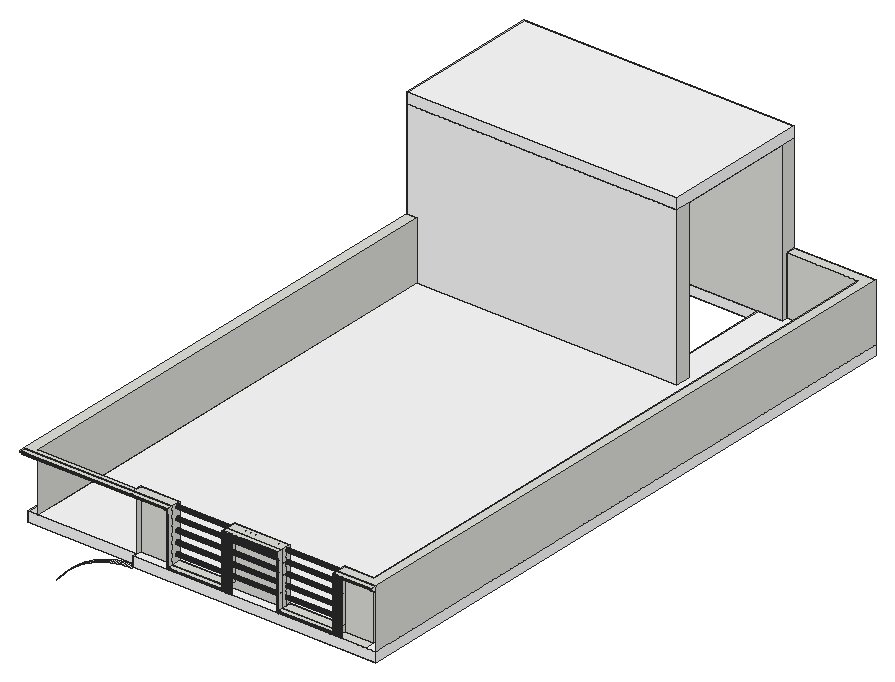
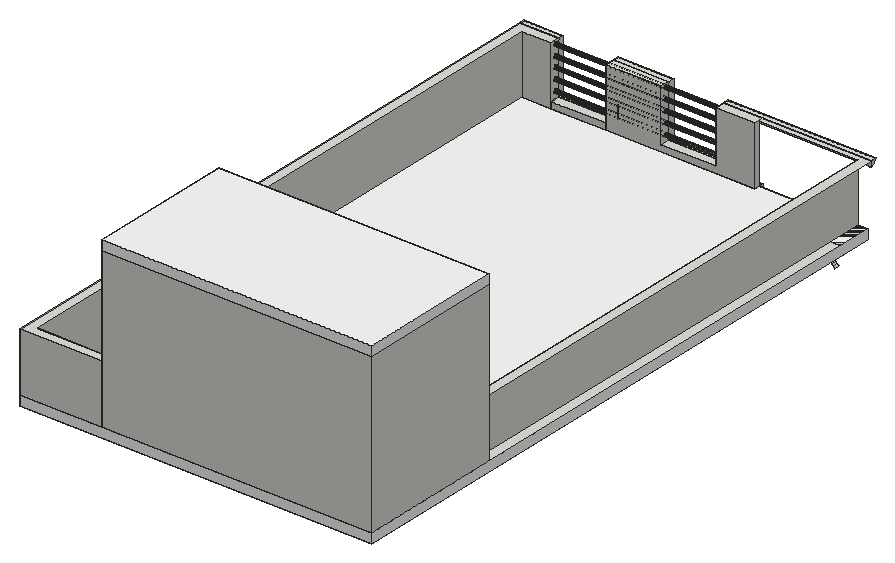
# SketchUp Ruby script. Lengths in inches.
U = 1.inch
M = Sketchup.active_model
def pt(a) = Geom::Point3d.new(a.map { |v| v * U })
def face(e, loops, mat)
  f = e.add_face(loops[0].map { |a| pt(a) })
  loops[1..].each { |l| e.add_face(l.map { |a| pt(a) }).erase! }
  f.material = f.back_material = mat if mat
  f
end
# faces: each face lists its corners as indices into pts; further lists are holes
def faces(e, pts, list, mat = nil) = list.each { |f| face(e, (f[0].is_a?(Array) ? f : [f]).map { |l| l.map { |i| pts[i] } }, mat) }
# xy, xz, yz: faces in a plane at the given z, y or x. An outline is a flat list of corners, or four numbers for a rectangle; further outlines are holes
def ring(l) = l.size == 4 ? [[l[0], l[1]], [l[2], l[1]], [l[2], l[3]], [l[0], l[3]]] : l.each_slice(2).to_a
def flat(e, list, mat, &to3) = list.each { |f| face(e, (f[0].is_a?(Array) ? f : [f]).map { |l| ring(l).map { |u, v| to3.(u, v) } }, mat) }
def xy(e, z, list, mat = nil) = flat(e, list, mat) { |x, y| [x, y, z] }
def xz(e, y, list, mat = nil) = flat(e, list, mat) { |x, z| [x, y, z] }
def yz(e, x, list, mat = nil) = flat(e, list, mat) { |y, z| [x, y, z] }
def lines(e, pts, list) = list.each { |a, b| e.add_line(pt(pts[a]), pt(pts[b])) }
# prism: a flat outline (further loops are holes) pulled along v
def prism(e, loops, v, mat = nil)
  f = face(e, loops, mat); d = Geom::Vector3d.new(v.map { |x| x * U })
  f.pushpull(f.normal.samedirection?(d) ? d.length : -d.length)
end
def box(e, o, s, mat = nil) = prism(e, [[o, [o[0] + s[0], o[1], o[2]], [o[0] + s[0], o[1] + s[1], o[2]], [o[0], o[1] + s[1], o[2]]]], [0, 0, s[2]], mat)
def at(x, y, z, deg = 0) = Geom::Transformation.translation(pt([x, y, z])) * Geom::Transformation.rotation(ORIGIN, Z_AXIS, deg.degrees)
def axes(o, x, y, z) = Geom::Transformation.new([*x, 0, *y, 0, *z, 0, *pt(o).to_a, 1])
def part(name) = M.definitions.add(name)
# library, detail: a bought-in or finely detailed component or shape, given as its bounding box
def library(name, o, s) = part(name).tap { |d| box(d.entities, o, s) }
def detail(e, o, s) = box(e.add_group.entities, o, s)
def put(e, d, t, mat = nil) = e.add_instance(d, t).tap { |i| i.material = mat if mat }
def group(e, t, mat = nil) = e.add_group.tap { |g| g.transformation = t; g.material = mat if mat }.entities
root = M.entities
M.materials.add("Leather White 002 15.0cm").color = [255, 255, 255]
M.materials.add("Manhattan Creative Coating ML 1016B 24.75cm").color = [255, 255, 255]
M.materials.add("Napura - nsi3013 29.32cm").color = [255, 255, 255]
M.materials.add("Steel Blurry").color = [182, 192, 192]
M.materials.add("T8600 Mosaic plaster 1019 34.05cm").color = [255, 255, 255]
c1 = part("Vertical post")
prism(c1.entities,[[[0.67,1.9375,0],[0.73,1.96,0],[0.99,2,0],[1.25,1.97,0],[1.49,1.87,0],[1.7,1.72,0],[1.86,1.51,0],[1.96,1.27,0],[2,1.01,0],[1.97,0.75,0],[1.87,0.51,0],[1.72,0.3,0],[1.51,0.14,0],[1.27,0.04,0],[1.01,0,0],[0.75,0.03,0],[0.67,0.0625,0],[0.51,0.13,0],[0.3,0.28,0],[0.14,0.49,0],[0.04,0.73,0],[0,0.99,0],[0.03,1.25,0],[0.13,1.49,0],[0.28,1.7,0],[0.49,1.86,0]]],[0,0,101.21])
xy(root,373.99,[[192.8125,53.93,213,54.62]])
xy(root,378,[[66.79,50.93,158.4,56.93],[158.4,50.93,192,56.93],[210,50.93,210,428.93,165.875,428.93,165.875,434.93,216,434.93,216,50.93],[192,50.93,210,56.93],[0,53.93,6,74.93],
  [0,74.93,6,344.93],[0,344.93,0,434.93,165.875,434.93,165.875,425.93,9,425.93,9,353.93,165.875,353.93,165.875,344.93]])
xy(root,378.5,[[87.54,50.68,127.65,50.93],[155.15,50.68,195.25,50.93]],"T8600 Mosaic plaster 1019 34.05cm")
xy(root,379.42,[[88.46,49.9,88.47,50,126.72,50,126.73,49.9],[156.0625,49.9,156.07,50,194.33,50,194.33,49.9],[88.47,50,88.46,50.09,126.73,50.09,126.72,50],[156.07,50,194.33,50.09]],"T8600 Mosaic plaster 1019 34.05cm")
xy(root,379.54,[[88.59,49.77,126.61,49.9],[156.1875,49.77,194.21,49.9]],"T8600 Mosaic plaster 1019 34.05cm")
xy(root,381.5,[[90.54,47.57,124.65,47.85],[158.15,47.57,192.25,47.85]])
xy(root,381.75,[[90.79,47.57,124.4,50.93],[158.4,47.57,192,50.93],[90.79,50.93,124.4,56.93],[158.4,50.93,192,56.93]])
xy(root,410.75,[[0,50.68,87.54,50.93],[127.65,50.68,127.65,50.93,155.15,50.68],[155.15,50.68,127.65,50.93,155.15,50.93],[195.25,50.68,216,50.93]],"T8600 Mosaic plaster 1019 34.05cm")
xy(root,411.67,[[0,49.9,0,50,88.47,50,88.46,49.9],[126.73,49.9,126.72,50,156.07,50,156.0625,49.9],[194.33,49.9,216,50],[0,50,0,50.09,88.46,50.09,88.47,50],[126.72,50,126.73,50.09,156.07,50.09,156.07,50],
  [194.33,50,216,50.09]],"T8600 Mosaic plaster 1019 34.05cm")
xy(root,411.79,[[0,49.77,88.59,49.9],[126.61,49.77,156.1875,49.9],[194.21,49.77,216,49.9]],"T8600 Mosaic plaster 1019 34.05cm")
xy(root,413.75,[[0,47.57,90.54,47.85],[124.65,47.57,158.15,47.85],[192.25,47.57,216,47.85]])
xy(root,414,[[0,47.57,90.79,50.93],[124.4,47.57,158.4,50.93],[192,47.57,216,50.93],[0,50.93,66.79,50.93,66.79,53.93,6,53.93,6,344.93,0,344.93],[66.79,50.93,90.79,56.93],
  [124.4,50.93,158.4,56.93],[192,50.93,216,50.93,216,434.93,165.875,434.93,165.875,428.93,210,428.93,210,56.93,192,56.93]])
xy(root,474.5625,[[0,344.93,165.875,353.93],[0,353.93,9,425.93],[9,353.93,165.875,425.93],[0,425.93,165.875,434.93]])
xy(root,481,[[0,344.93,165.875,434.93]],"Napura - nsi3013 29.32cm")
xz(root,47.57,[[90.54,381.5,124.65,381.5,124.65,413.75,158.15,413.75,158.15,381.5,192.25,381.5,192.25,413.75,216,413.75,216,414,192,414,192,381.75,158.4,381.75,158.4,414,124.4,414,124.4,381.75,90.79,381.75,90.79,414,0,414,0,413.75,90.54,413.75]],"T8600 Mosaic plaster 1019 34.05cm")
xz(root,47.85,[[90.34,381.29,124.85,381.29,124.85,413.54,157.94,413.54,157.94,381.29,192.46,381.29,192.46,413.54,216,413.54,216,413.75,192.25,413.75,192.25,381.5,158.15,381.5,158.15,413.75,124.65,413.75,124.65,381.5,90.54,381.5,90.54,413.75,0,413.75,0,413.54,90.34,413.54]],"T8600 Mosaic plaster 1019 34.05cm")
xz(root,49.9,[[88.46,379.42,126.73,379.42,126.73,411.67,156.0625,411.67,156.0625,379.42,194.33,379.42,194.33,411.67,216,411.67,216,411.79,194.21,411.79,194.21,379.54,156.1875,379.54,156.1875,411.79,126.61,411.79,126.61,379.54,88.59,379.54,88.59,411.79,0,411.79,0,411.67,88.46,411.67]],"T8600 Mosaic plaster 1019 34.05cm")
xz(root,50.68,[[87.54,378.5,127.65,378.5,127.65,410.75,155.15,410.75,155.15,378.5,195.25,378.5,195.25,410.75,216,410.75,216,411,195,411,195,378.75,155.4,378.75,155.4,411,127.4,411,127.4,378.75,87.79,378.75,87.79,411,0,411,0,410.75,87.54,410.75],[87.79,378.75,127.4,378.75,127.3,378.85,87.89,378.85],[87.79,378.75,87.89,378.85,87.89,411.1,87.79,411],[127.4,378.75,127.4,411,127.3,411.1,127.3,378.85],[155.4,378.75,155.49,378.85,155.49,411.1,155.4,411],
  [155.4,378.75,195,378.75,194.9,378.85,155.49,378.85],[195,378.75,195,411,194.9,411.1,194.9,378.85],[0,411,87.79,411,87.89,411.1,0,411.1],[127.4,411,155.4,411,155.49,411.1,127.3,411.1],[195,411,216,411,216,411.1,194.9,411.1]],"T8600 Mosaic plaster 1019 34.05cm")
xz(root,50.93,[[87.54,378.5,127.65,378.5,127.65,410.75,155.15,410.75,155.15,378.5,195.25,378.5,195.25,410.75,216,410.75,216,414,192,414,192,381.75,158.4,381.75,158.4,414,124.4,414,124.4,381.75,90.79,381.75,90.79,414,0,414,0,410.75,87.54,410.75]])
xz(root,56.93,[[66.79,378,66.79,414,90.79,414,90.79,381.75,124.4,381.75,124.4,414,158.4,414,158.4,378],[158.4,378,192,381.75],[192,378,210,414]])
xz(root,344.93,[[0,378,6,414]])
xz(root,344.93,[[6,378,165.875,378,165.875,474.5625,0,474.5625,0,414,6,414],[0,474.5625,165.875,481]],"Napura - nsi3013 29.32cm")
xz(root,353.93,[[9,378,165.875,474.5625]])
xz(root,425.93,[[9,378,165.875,474.5625]])
xz(root,428.93,[[165.875,378,210,414]])
xz(root,434.93,[[0,378,165.875,474.5625],[165.875,378,216,414]])
xz(root,434.93,[[0,474.5625,165.875,481]],"Napura - nsi3013 29.32cm")
yz(root,0,[[344.93,378,434.93,474.5625],[50.68,410.75,50.68,411.1,50.62,411.28,50.57,411.37,50.51,411.45,50.37,411.57,50.28,411.62,50.1875,411.65,50.09,411.67,49.9,411.67,49.9,411.79,49.77,411.79,49.67,411.8,49.57,411.8125,49.48,411.84,49.38,411.88,49.3,411.93,49.21,411.99,49.07,412.13,48.97,412.31,48.93,412.4,48.91,412.5,48.875,412.625,48.83,412.75,48.77,412.87,48.7,412.98,48.625,413.08,48.54,413.18,48.4375,413.27,48.33,413.34,48.22,413.41,48.1,413.47,47.98,413.51,47.85,413.54,47.85,413.75,47.57,413.75,47.57,414,50.93,414,50.93,410.75]])
yz(root,0,[[344.93,474.5625,434.93,481]],"Napura - nsi3013 29.32cm")
yz(root,6,[[53.93,378,344.93,414]])
yz(root,9,[[353.93,378,425.93,474.5625]])
yz(root,66.79,[[50.93,371.45,53.93,378],[53.93,378,56.93,414]])
yz(root,87.54,[[50.68,378.5,50.93,410.75]],"T8600 Mosaic plaster 1019 34.05cm")
yz(root,88.59,[[49.77,379.54,49.67,379.55,49.67,411.8,49.77,411.79],[49.77,379.54,49.9,411.79]],"T8600 Mosaic plaster 1019 34.05cm")
yz(root,90.54,[[47.57,381.5,47.85,413.75]])
yz(root,90.79,[[47.57,381.75,50.93,414],[50.93,381.75,56.93,414]])
yz(root,124.4,[[47.57,381.75,50.93,414],[50.93,381.75,56.93,414]])
yz(root,124.65,[[47.57,381.5,47.85,413.75]])
yz(root,126.61,[[49.77,379.54,49.9,411.79]],"T8600 Mosaic plaster 1019 34.05cm")
yz(root,127.65,[[50.68,378.5,50.93,410.75]],"T8600 Mosaic plaster 1019 34.05cm")
yz(root,155.15,[[50.68,378.5,50.93,410.75]],"T8600 Mosaic plaster 1019 34.05cm")
yz(root,156.07,[[50,379.42,50.09,411.67]],"T8600 Mosaic plaster 1019 34.05cm")
yz(root,156.1875,[[49.77,379.54,49.9,411.79]],"T8600 Mosaic plaster 1019 34.05cm")
yz(root,158.15,[[47.57,381.5,47.85,413.75]])
yz(root,158.4,[[53.93,378,56.93,381.75],[47.57,381.75,50.93,414],[50.93,381.75,53.93,414],[53.93,381.75,56.93,414]])
yz(root,165.875,[[344.93,378,353.93,474.5625],[425.93,378,428.93,378,428.93,414,434.93,414,434.93,474.5625,425.93,474.5625],[428.93,378,434.93,414]])
yz(root,165.875,[[344.93,474.5625,434.93,481]],"Napura - nsi3013 29.32cm")
yz(root,192,[[53.93,378,56.93,381.75],[47.57,381.75,50.93,414],[50.93,381.75,56.93,414]])
yz(root,192.25,[[47.57,381.5,47.85,413.75]])
yz(root,194.21,[[49.77,379.54,49.9,411.79]],"T8600 Mosaic plaster 1019 34.05cm")
yz(root,194.33,[[49.9,379.42,50,411.67],[50,379.42,50.09,411.67]],"T8600 Mosaic plaster 1019 34.05cm")
yz(root,195.25,[[50.68,378.5,50.93,410.75]],"T8600 Mosaic plaster 1019 34.05cm")
yz(root,210,[[56.93,378,428.93,414]])
yz(root,216,[[50.93,378,434.93,414]])
yz(root,216,[[50.68,410.75,50.93,410.75,50.93,414,47.57,414,47.57,413.75,47.85,413.75,47.85,413.54,47.98,413.51,48.1,413.47,48.22,413.41,48.33,413.34,48.4375,413.27,48.54,413.18,48.625,413.08,48.7,412.98,48.77,412.87,48.83,412.75,48.875,412.625,48.91,412.5,48.93,412.4,48.97,412.31,49.07,412.13,49.21,411.99,49.3,411.93,49.38,411.88,49.48,411.84,49.57,411.8125,49.67,411.8,49.77,411.79,49.9,411.79,49.9,411.67,50.09,411.67,50.1875,411.65,50.28,411.62,50.37,411.57,50.51,411.45,50.57,411.37,50.62,411.28,50.68,411.1]],"T8600 Mosaic plaster 1019 34.05cm")
p = [[20.99,50.93,349.89],[20.21,50.93,348.93],[20.21,53.93,348.93],[20.99,53.93,349.89],[21.79,50.93,350.84],[21.79,53.93,350.84],
  [22.62,50.93,351.78],[22.62,53.93,351.78],[23.46,50.93,352.7],[23.46,53.93,352.7],[24.32,50.93,353.59],[24.32,53.93,353.59],
  [25.2,50.93,354.47],[25.2,53.93,354.47],[26.1,50.93,355.34],[26.1,53.93,355.34],[27.02,50.93,356.18],[27.02,53.93,356.18],
  [27.95,50.93,357],[27.95,53.93,357],[28.9,50.93,357.81],[28.9,53.93,357.81],[29.87,50.93,358.59],[29.87,53.93,358.59],
  [30.85,50.93,359.35],[30.85,53.93,359.35],[31.85,50.93,360.09],[31.85,53.93,360.09],[32.87,50.93,360.82],[32.87,53.93,360.82],
  [33.9,50.93,361.52],[33.9,53.93,361.52],[34.94,50.93,362.19],[34.94,53.93,362.19],[36,50.93,362.85],[36,53.93,362.85],
  [37.07,50.93,363.48],[37.07,53.93,363.48],[38.16,50.93,364.1],[38.16,53.93,364.1],[39.25,50.93,364.68],[39.25,53.93,364.68],
  [40.36,50.93,365.25],[40.36,53.93,365.25],[41.48,50.93,365.79],[41.48,53.93,365.79],[42.62,50.93,366.31],[42.62,53.93,366.31],
  [43.76,50.93,366.8],[43.76,53.93,366.8],[44.91,50.93,367.27],[44.91,53.93,367.27],[46.07,50.93,367.72],[46.07,53.93,367.72],
  [47.24,50.93,368.14],[47.24,53.93,368.14],[48.42,50.93,368.54],[48.42,53.93,368.54],[49.61,50.93,368.91],[49.61,53.93,368.91],
  [50.81,50.93,369.26],[50.81,53.93,369.26],[52.01,50.93,369.58],[52.01,53.93,369.58],[53.22,50.93,369.88],[53.22,53.93,369.88],
  [54.43,50.93,370.15],[54.43,53.93,370.15],[55.66,50.93,370.4],[55.66,53.93,370.4],[56.88,50.93,370.62],[56.88,53.93,370.62],
  [58.11,50.93,370.8125],[58.11,53.93,370.8125],[59.34,50.93,370.98],[59.34,53.93,370.98],[60.58,50.93,371.12],[60.58,53.93,371.12],
  [61.82,50.93,371.24],[61.82,53.93,371.24],[63.0625,50.93,371.33],[63.0625,53.93,371.33],[64.31,50.93,371.4],[64.31,53.93,371.4],
  [65.55,50.93,371.44],[65.55,53.93,371.44],[66.79,50.93,371.45],[66.79,53.93,371.45],[127.3,50.68,378.85],[127.21,50.65,378.94],
  [87.99,50.65,378.94],[87.89,50.68,378.85],[87.99,50.65,411.19],[87.89,50.68,411.1],[127.3,50.68,411.1],[127.21,50.65,411.19],
  [194.9,50.68,378.85],[194.81,50.65,378.94],[155.59,50.65,378.94],[155.49,50.68,378.85],[155.59,50.65,411.19],[155.49,50.68,411.1],
  [194.9,50.68,411.1],[194.81,50.65,411.19],[127.11,50.62,379.03],[88.08,50.62,379.03],[88.08,50.62,411.28],[127.11,50.62,411.28],
  [194.72,50.62,379.03],[155.68,50.62,379.03],[155.68,50.62,411.28],[194.72,50.62,411.28],[127.03,50.57,379.12],[88.16,50.57,379.12],
  [88.16,50.57,411.37],[127.03,50.57,411.37],[194.63,50.57,379.12],[155.77,50.57,379.12],[155.77,50.57,411.37],[194.63,50.57,411.37],
  [126.95,50.51,379.2],[88.24,50.51,379.2],[88.24,50.51,411.45],[126.95,50.51,411.45],[194.55,50.51,379.2],[155.84,50.51,379.2],
  [155.84,50.51,411.45],[194.55,50.51,411.45],[126.88,50.44,379.26],[88.31,50.44,379.26],[88.31,50.44,411.51],[126.88,50.44,411.51],
  [194.49,50.44,379.26],[155.91,50.44,379.26],[155.91,50.44,411.51],[194.49,50.44,411.51],[126.83,50.37,379.32],[126.78,50.28,379.37],
  [88.41,50.28,379.37],[88.37,50.37,379.32],[88.41,50.28,411.62],[88.37,50.37,411.57],[126.83,50.37,411.57],[126.78,50.28,411.62],
  [194.43,50.37,379.32],[194.38,50.28,379.37],[156.01,50.28,379.37],[155.97,50.37,379.32],[156.01,50.28,411.62],[155.97,50.37,411.57],
  [194.43,50.37,411.57],[194.38,50.28,411.62],[88.47,50,379.42],[88.46,49.9,379.42],[88.46,49.9,411.67],[88.47,50,411.67],
  [126.72,50,411.67],[126.73,49.9,411.67],[126.73,49.9,379.42],[126.72,50,379.42],[156.07,50,379.42],[156.0625,49.9,379.42],
  [156.0625,49.9,411.67],[156.07,50,411.67],[88.46,50.09,379.42],[88.46,50.09,411.67],[126.73,50.09,411.67],[126.73,50.09,379.42],
  [126.75,50.1875,379.4],[88.44,50.1875,379.4],[88.44,50.1875,411.65],[126.75,50.1875,411.65],[194.35,50.1875,379.4],[194.33,50.09,379.42],
  [156.07,50.09,379.42],[156.05,50.1875,379.4],[156.07,50.09,411.67],[156.05,50.1875,411.65],[194.35,50.1875,411.65],[194.33,50.09,411.67],
  [126.6,49.67,379.55],[126.58,49.57,379.5625],[88.61,49.57,379.5625],[88.59,49.67,379.55],[88.61,49.57,411.8125],[88.59,49.67,411.8],
  [126.6,49.67,411.8],[126.58,49.57,411.8125],[194.2,49.67,379.55],[194.1875,49.57,379.5625],[156.21,49.57,379.5625],[156.19,49.67,379.55],
  [156.21,49.57,411.8125],[156.19,49.67,411.8],[194.2,49.67,411.8],[194.1875,49.57,411.8125],[126.61,49.77,379.54],[88.59,49.77,379.54],
  [126.61,49.77,411.79],[194.21,49.77,379.54],[156.1875,49.77,379.54],[156.1875,49.77,411.79],[194.21,49.77,411.79],[126.52,49.38,379.63],
  [126.47,49.3,379.68],[88.73,49.3,379.68],[88.68,49.38,379.63],[88.73,49.3,411.93],[88.68,49.38,411.88],[126.52,49.38,411.88],
  [126.47,49.3,411.93],[194.12,49.38,379.63],[194.07,49.3,379.68],[156.33,49.3,379.68],[156.28,49.38,379.63],[156.33,49.3,411.93],
  [156.28,49.38,411.88],[194.12,49.38,411.88],[194.07,49.3,411.93],[126.56,49.48,379.59],[88.64,49.48,379.59],[88.64,49.48,411.84],
  [126.56,49.48,411.84],[194.16,49.48,379.59],[156.24,49.48,379.59],[156.24,49.48,411.84],[194.16,49.48,411.84],[126.41,49.21,379.74],
  [126.34,49.14,379.81],[88.85,49.14,379.81],[88.78,49.21,379.74],[88.85,49.14,412.06],[88.78,49.21,411.99],[126.41,49.21,411.99],
  [126.34,49.14,412.06],[194.01,49.21,379.74],[193.94,49.14,379.81],[156.45,49.14,379.81],[156.39,49.21,379.74],[156.45,49.14,412.06],
  [156.39,49.21,411.99],[194.01,49.21,411.99],[193.94,49.14,412.06],[126.26,49.07,379.88],[88.93,49.07,379.88],[88.93,49.07,412.13],
  [126.26,49.07,412.13],[193.87,49.07,379.88],[156.53,49.07,379.88],[156.53,49.07,412.13],[193.87,49.07,412.13],[126.18,49.02,379.97],
  [89.01,49.02,379.97],[89.01,49.02,412.22],[126.18,49.02,412.22],[193.78,49.02,379.97],[156.61,49.02,379.97],[156.61,49.02,412.22],
  [193.78,49.02,412.22],[126.09,48.97,380.06],[89.1,48.97,380.06],[89.1,48.97,412.31],[126.09,48.97,412.31],[193.69,48.97,380.06],
  [156.7,48.97,380.06],[156.7,48.97,412.31],[193.69,48.97,412.31],[126,48.93,380.15],[89.19,48.93,380.15],[89.19,48.93,412.4],
  [125.9,48.91,380.25],[89.29,48.91,380.25],[89.29,48.91,412.5],[126,48.93,412.4],[125.9,48.91,412.5],[193.6,48.93,380.15],
  [156.8,48.93,380.15],[156.8,48.93,412.4],[193.5,48.91,380.25],[156.89,48.91,380.25],[156.89,48.91,412.5],[193.6,48.93,412.4],
  [193.5,48.91,412.5],[125.77,48.875,380.375],[89.42,48.875,380.375],[89.42,48.875,412.625],[125.77,48.875,412.625],[193.375,48.875,380.375],
  [157.02,48.875,380.375],[157.02,48.875,412.625],[193.375,48.875,412.625],[125.65,48.83,380.5],[89.54,48.83,380.5],[89.54,48.83,412.75],
  [125.65,48.83,412.75],[193.25,48.83,380.5],[157.14,48.83,380.5],[157.14,48.83,412.75],[193.25,48.83,412.75],[125.53,48.77,380.62],
  [89.66,48.77,380.62],[89.66,48.77,412.87],[125.53,48.77,412.87],[193.13,48.77,380.62],[157.26,48.77,380.62],[157.26,48.77,412.87],
  [193.13,48.77,412.87],[125.42,48.7,380.73],[89.77,48.7,380.73],[89.77,48.7,412.98],[125.42,48.7,412.98],[193.02,48.7,380.73],
  [157.375,48.7,380.73],[157.375,48.7,412.98],[193.02,48.7,412.98],[125.32,48.625,380.83],[89.88,48.625,380.83],[89.88,48.625,413.08],
  [125.32,48.625,413.08],[192.92,48.625,380.83],[157.48,48.625,380.83],[157.48,48.625,413.08],[192.92,48.625,413.08],[125.22,48.54,380.93],
  [89.97,48.54,380.93],[89.97,48.54,413.18],[125.22,48.54,413.18],[192.82,48.54,380.93],[157.58,48.54,380.93],[157.58,48.54,413.18],
  [192.82,48.54,413.18],[125.13,48.4375,381.02],[90.0625,48.4375,381.02],[90.0625,48.4375,413.27],[125.13,48.4375,413.27],[192.73,48.4375,381.02],
  [157.66,48.4375,381.02],[157.66,48.4375,413.27],[192.73,48.4375,413.27],[125.05,48.33,381.09],[90.14,48.33,381.09],[90.14,48.33,413.34],
  [125.05,48.33,413.34],[192.66,48.33,381.09],[157.74,48.33,381.09],[157.74,48.33,413.34],[192.66,48.33,413.34],[124.99,48.22,381.16],
  [90.21,48.22,381.16],[90.21,48.22,413.41],[124.99,48.22,413.41],[192.59,48.22,381.16],[157.81,48.22,381.16],[157.81,48.22,413.41],
  [192.59,48.22,413.41],[124.93,48.1,381.22],[124.89,47.98,381.26],[90.31,47.98,381.26],[90.26,48.1,381.22],[90.31,47.98,413.51],
  [90.26,48.1,413.47],[124.93,48.1,413.47],[124.89,47.98,413.51],[192.53,48.1,381.22],[192.49,47.98,381.26],[157.91,47.98,381.26],
  [157.86,48.1,381.22],[157.91,47.98,413.51],[157.86,48.1,413.47],[192.53,48.1,413.47],[192.49,47.98,413.51],[124.85,47.85,381.29],
  [90.34,47.85,381.29],[90.34,47.85,413.54],[124.85,47.85,413.54],[192.46,47.85,381.29],[157.94,47.85,381.29],[157.94,47.85,413.54],
  [192.46,47.85,413.54],[66.79,50.65,411.19],[0,50.65,411.19],[0,50.68,411.1],[66.79,50.68,411.1],[216,50.68,411.1],
  [216,50.65,411.19],[66.79,50.62,411.28],[0,50.62,411.28],[216,50.62,411.28],[66.79,50.57,411.37],[0,50.57,411.37],
  [216,50.57,411.37],[66.79,50.44,411.51],[0,50.44,411.51],[0,50.51,411.45],[66.79,50.51,411.45],[216,50.51,411.45],
  [216,50.44,411.51],[66.79,50.37,411.57],[0,50.37,411.57],[216,50.37,411.57],[66.79,50.09,411.67],[0,50.09,411.67],
  [0,50.1875,411.65],[66.79,50.1875,411.65],[216,50.1875,411.65],[216,50.09,411.67],[0,50.28,411.62],[66.79,50.28,411.62],
  [216,50.28,411.62],[66.79,49.38,411.88],[0,49.38,411.88],[0,49.48,411.84],[66.79,49.48,411.84],[216,49.48,411.84],
  [216,49.38,411.88],[0,49.57,411.8125],[66.79,49.57,411.8125],[216,49.57,411.8125],[0,49.67,411.8],[66.79,49.67,411.8],
  [216,49.67,411.8],[88.59,49.77,411.79],[0,49.77,411.79],[66.79,49.77,411.79],[216,49.77,411.79],[66.79,49.21,411.99],
  [0,49.21,411.99],[0,49.3,411.93],[66.79,49.3,411.93],[216,49.3,411.93],[216,49.21,411.99],[66.79,49.14,412.06],
  [0,49.14,412.06],[216,49.14,412.06],[66.79,49.02,412.22],[0,49.02,412.22],[0,49.07,412.13],[66.79,49.07,412.13],
  [216,49.07,412.13],[216,49.02,412.22],[66.79,48.97,412.31],[0,48.97,412.31],[216,48.97,412.31],[66.79,48.93,412.4],
  [0,48.93,412.4],[216,48.93,412.4],[66.79,48.91,412.5],[0,48.91,412.5],[216,48.91,412.5],[66.79,48.875,412.625],
  [0,48.875,412.625],[216,48.875,412.625],[66.79,48.83,412.75],[0,48.83,412.75],[216,48.83,412.75],[66.79,48.77,412.87],
  [0,48.77,412.87],[216,48.77,412.87],[66.79,48.7,412.98],[0,48.7,412.98],[216,48.7,412.98],[66.79,48.625,413.08],
  [0,48.625,413.08],[216,48.625,413.08],[66.79,48.54,413.18],[0,48.54,413.18],[216,48.54,413.18],[66.79,48.4375,413.27],
  [0,48.4375,413.27],[216,48.4375,413.27],[66.79,48.22,413.41],[0,48.22,413.41],[0,48.33,413.34],[66.79,48.33,413.34],
  [216,48.33,413.34],[216,48.22,413.41],[66.79,48.1,413.47],[0,48.1,413.47],[216,48.1,413.47],[66.79,47.85,413.54],
  [0,47.85,413.54],[0,47.98,413.51],[66.79,47.98,413.51],[216,47.98,413.51],[216,47.85,413.54],[155.15,50.68,378.5],
  [127.65,50.93,378.5]]
faces(root,p,[[0,1,2,3],[4,0,3,5],[6,4,5,7],[8,6,7,9],[10,8,9,11],[12,10,11,13],[14,12,13,15],[16,14,15,17],
  [18,16,17,19],[20,18,19,21],[22,20,21,23],[24,22,23,25],[26,24,25,27],[28,26,27,29],[30,28,29,31],[32,30,31,33],
  [34,32,33,35],[36,34,35,37],[38,36,37,39],[40,38,39,41],[42,40,41,43],[44,42,43,45],[46,44,45,47],[48,46,47,49],
  [50,48,49,51],[52,50,51,53],[54,52,53,55],[56,54,55,57],[58,56,57,59],[60,58,59,61],[62,60,61,63],[64,62,63,65],
  [66,64,65,67],[68,66,67,69],[70,68,69,71],[72,70,71,73],[74,72,73,75],[76,74,75,77],[78,76,77,79],[80,78,79,81],
  [82,80,81,83],[84,82,83,85],[86,84,85,87]],"Leather White 002 15.0cm")
faces(root,p,[[88,89,90,91],[91,90,92,93],[94,95,89,88],[96,97,98,99],[99,98,100,101],[102,103,97,96],[89,104,105,90],[90,105,106,92],
  [95,107,104,89],[97,108,109,98],[98,109,110,100],[103,111,108,97],[104,112,113,105],[105,113,114,106],[107,115,112,104],[108,116,117,109],
  [109,117,118,110],[111,119,116,108],[112,120,121,113],[113,121,122,114],[115,123,120,112],[116,124,125,117],[117,125,126,118],[119,127,124,116],
  [120,128,129,121],[121,129,130,122],[123,131,128,120],[124,132,133,125],[125,133,134,126],[127,135,132,124],[136,137,138,139],[139,138,140,141],
  [142,143,137,136],[144,145,146,147],[147,146,148,149],[150,151,145,144],[128,136,139,129],[129,139,141,130],[131,142,136,128],[132,144,147,133],
  [133,147,149,134],[135,150,144,132],[152,153,154,155],[156,157,158,159],[160,161,162,163],[164,152,155,165],[166,156,159,167],[168,167,164,169],
  [169,164,165,170],[171,166,167,168],[172,173,174,175],[175,174,176,177],[178,179,173,172],[137,168,169,138],[138,169,170,140],[143,171,168,137],
  [145,172,175,146],[146,175,177,148],[151,178,172,145],[180,181,182,183],[183,182,184,185],[186,187,181,180],[188,189,190,191],[191,190,192,193],
  [194,195,189,188],[196,180,183,197],[198,186,180,196],[199,188,191,200],[200,191,193,201],[202,194,188,199],[203,204,205,206],[206,205,207,208],
  [209,210,204,203],[211,212,213,214],[214,213,215,216],[217,218,212,211],[219,203,206,220],[220,206,208,221],[222,209,203,219],[223,211,214,224],
  [224,214,216,225],[226,217,211,223],[181,219,220,182],[182,220,221,184],[187,222,219,181],[189,223,224,190],[190,224,225,192],[195,226,223,189],
  [227,228,229,230],[230,229,231,232],[233,234,228,227],[235,236,237,238],[238,237,239,240],[241,242,236,235],[204,227,230,205],[205,230,232,207],
  [210,233,227,204],[212,235,238,213],[213,238,240,215],[218,241,235,212],[228,243,244,229],[229,244,245,231],[234,246,243,228],[236,247,248,237],
  [237,248,249,239],[242,250,247,236],[243,251,252,244],[244,252,253,245],[246,254,251,243],[247,255,256,248],[248,256,257,249],[250,258,255,247],
  [251,259,260,252],[252,260,261,253],[254,262,259,251],[255,263,264,256],[256,264,265,257],[258,266,263,255],[259,267,268,260],[260,268,269,261],
  [267,270,271,268],[268,271,272,269],[273,274,270,267],[262,273,267,259],[263,275,276,264],[264,276,277,265],[275,278,279,276],[276,279,280,277],
  [281,282,278,275],[266,281,275,263],[270,283,284,271],[271,284,285,272],[274,286,283,270],[278,287,288,279],[279,288,289,280],[282,290,287,278],
  [283,291,292,284],[284,292,293,285],[286,294,291,283],[287,295,296,288],[288,296,297,289],[290,298,295,287],[291,299,300,292],[292,300,301,293],
  [294,302,299,291],[295,303,304,296],[296,304,305,297],[298,306,303,295],[299,307,308,300],[300,308,309,301],[302,310,307,299],[303,311,312,304],
  [304,312,313,305],[306,314,311,303],[307,315,316,308],[308,316,317,309],[310,318,315,307],[311,319,320,312],[312,320,321,313],[314,322,319,311],
  [315,323,324,316],[316,324,325,317],[318,326,323,315],[319,327,328,320],[320,328,329,321],[322,330,327,319],[323,331,332,324],[324,332,333,325],
  [326,334,331,323],[327,335,336,328],[328,336,337,329],[330,338,335,327],[331,339,340,332],[332,340,341,333],[334,342,339,331],[335,343,344,336],
  [336,344,345,337],[338,346,343,335],[339,347,348,340],[340,348,349,341],[342,350,347,339],[343,351,352,344],[344,352,353,345],[346,354,351,343],
  [355,356,357,358],[358,357,359,360],[361,362,356,355],[363,364,365,366],[366,365,367,368],[369,370,364,363],[347,355,358,348],[348,358,360,349],
  [350,361,355,347],[351,363,366,352],[352,366,368,353],[354,369,363,351],[356,371,372,357],[357,372,373,359],[362,374,371,356],[364,375,376,365],
  [365,376,377,367],[370,378,375,364],[93,92,379,380,381,382],[101,100,95,94],[383,384,103,102],[92,106,385,386,380,379],[100,110,107,95],[384,387,111,103],
  [106,114,388,389,386,385],[110,118,115,107],[387,390,119,111],[122,130,391,392,393,394],[126,134,131,123],[395,396,135,127],[114,122,394,393,389,388],[118,126,123,115],
  [390,395,127,119],[130,141,397,398,392,391],[134,149,142,131],[396,399,150,135],[170,165,400,401,402,403],[177,176,166,171],[404,405,179,178],[140,170,403,402,406,407],
  [148,177,171,143],[408,404,178,151],[141,140,407,406,398,397],[149,148,143,142],[399,408,151,150],[221,208,409,410,411,412],[225,216,209,222],[413,414,217,226],
  [184,221,412,411,415,416],[192,225,222,187],[417,413,226,195],[185,184,416,415,418,419],[193,192,187,186],[420,417,195,194],[421,185,419,418,422,423],[201,193,186,198],
  [424,420,194,202],[207,232,425,426,427,428],[215,240,233,210],[429,430,241,218],[208,207,428,427,410,409],[216,215,210,209],[414,429,218,217],[232,231,431,432,426,425],
  [240,239,234,233],[430,433,242,241],[245,253,434,435,436,437],[249,257,254,246],[438,439,258,250],[231,245,437,436,432,431],[239,249,246,234],[433,438,250,242],
  [253,261,440,441,435,434],[257,265,262,254],[439,442,266,258],[261,269,443,444,441,440],[265,277,273,262],[442,445,281,266],[269,272,446,447,444,443],[277,280,274,273],
  [445,448,282,281],[272,285,449,450,447,446],[280,289,286,274],[448,451,290,282],[285,293,452,453,450,449],[289,297,294,286],[451,454,298,290],[293,301,455,456,453,452],
  [297,305,302,294],[454,457,306,298],[301,309,458,459,456,455],[305,313,310,302],[457,460,314,306],[309,317,461,462,459,458],[313,321,318,310],[460,463,322,314],
  [317,325,464,465,462,461],[321,329,326,318],[463,466,330,322],[325,333,467,468,465,464],[329,337,334,326],[466,469,338,330],[341,349,470,471,472,473],[345,353,350,342],
  [474,475,354,346],[333,341,473,472,468,467],[337,345,342,334],[469,474,346,338],[349,360,476,477,471,470],[353,368,361,350],[475,478,369,354],[359,373,479,480,481,482],
  [367,377,374,362],[483,484,378,370],[360,359,482,481,477,476],[368,367,362,361],[478,483,370,369]],"T8600 Mosaic plaster 1019 34.05cm")
lines(root,p,[[485,486]])
g1 = group(root,at(0,74.93,372),"Manhattan Creative Coating ML 1016B 24.75cm")
prism(g1,[[[216,360,0],[216,-24,0],[66.79,-24,0],[66.79,-21,0],[0,-21,0],[0,360,0]],[[151,279,0],[151,351,0],[9,351,0],[9,279,0]]],[0,0,6])
put(root,c1,axes([90.79,53.26,385.43],[0,1,0],[0,0,1],[1,0,0]),"Steel Blurry")
put(root,c1,axes([90.79,53.26,391.97],[0,1,0],[0,0,1],[1,0,0]),"Steel Blurry")
put(root,c1,axes([90.79,53.26,398.5],[0,1,0],[0,0,1],[1,0,0]),"Steel Blurry")
put(root,c1,axes([90.79,53.26,405.03],[0,1,0],[0,0,1],[1,0,0]),"Steel Blurry")
put(root,c1,axes([90.79,53.26,411.56],[0,1,0],[0,0,1],[1,0,0]),"Steel Blurry")
